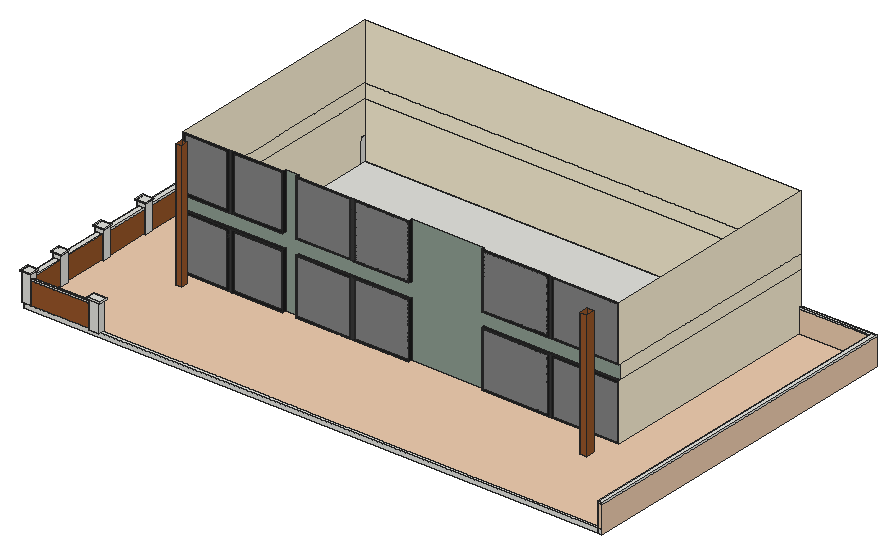
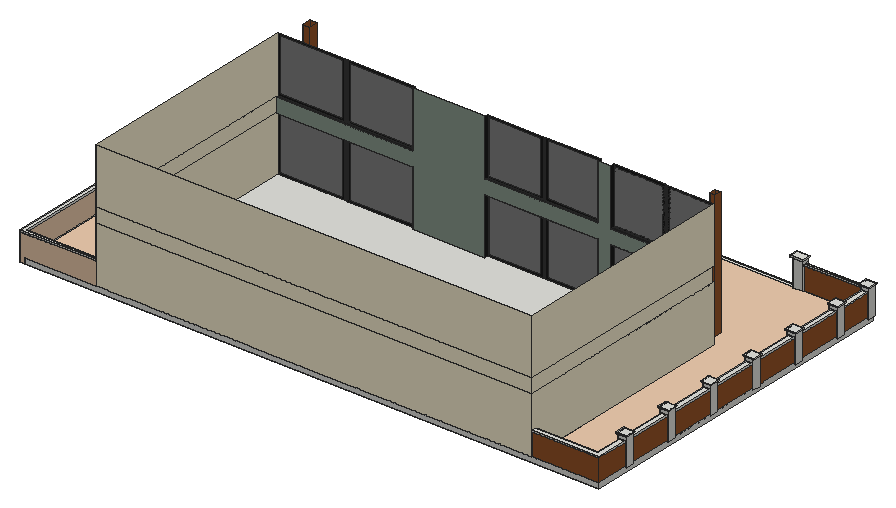
# SketchUp Ruby script. Lengths in inches.
U = 1.inch
M = Sketchup.active_model
def pt(a) = Geom::Point3d.new(a.map { |v| v * U })
def face(e, loops, mat)
  f = e.add_face(loops[0].map { |a| pt(a) })
  loops[1..].each { |l| e.add_face(l.map { |a| pt(a) }).erase! }
  f.material = f.back_material = mat if mat
  f
end
# faces: each face lists its corners as indices into pts; further lists are holes
def faces(e, pts, list, mat = nil) = list.each { |f| face(e, (f[0].is_a?(Array) ? f : [f]).map { |l| l.map { |i| pts[i] } }, mat) }
# xy, xz, yz: faces in a plane at the given z, y or x. An outline is a flat list of corners, or four numbers for a rectangle; further outlines are holes
def ring(l) = l.size == 4 ? [[l[0], l[1]], [l[2], l[1]], [l[2], l[3]], [l[0], l[3]]] : l.each_slice(2).to_a
def flat(e, list, mat, &to3) = list.each { |f| face(e, (f[0].is_a?(Array) ? f : [f]).map { |l| ring(l).map { |u, v| to3.(u, v) } }, mat) }
def xy(e, z, list, mat = nil) = flat(e, list, mat) { |x, y| [x, y, z] }
def xz(e, y, list, mat = nil) = flat(e, list, mat) { |x, z| [x, y, z] }
def yz(e, x, list, mat = nil) = flat(e, list, mat) { |y, z| [x, y, z] }
def lines(e, pts, list) = list.each { |a, b| e.add_line(pt(pts[a]), pt(pts[b])) }
# prism: a flat outline (further loops are holes) pulled along v
def prism(e, loops, v, mat = nil)
  f = face(e, loops, mat); d = Geom::Vector3d.new(v.map { |x| x * U })
  f.pushpull(f.normal.samedirection?(d) ? d.length : -d.length)
end
def box(e, o, s, mat = nil) = prism(e, [[o, [o[0] + s[0], o[1], o[2]], [o[0] + s[0], o[1] + s[1], o[2]], [o[0], o[1] + s[1], o[2]]]], [0, 0, s[2]], mat)
def at(x, y, z, deg = 0) = Geom::Transformation.translation(pt([x, y, z])) * Geom::Transformation.rotation(ORIGIN, Z_AXIS, deg.degrees)
def axes(o, x, y, z) = Geom::Transformation.new([*x, 0, *y, 0, *z, 0, *pt(o).to_a, 1])
def part(name) = M.definitions.add(name)
# library, detail: a bought-in or finely detailed component or shape, given as its bounding box
def library(name, o, s) = part(name).tap { |d| box(d.entities, o, s) }
def detail(e, o, s) = box(e.add_group.entities, o, s)
def put(e, d, t, mat = nil) = e.add_instance(d, t).tap { |i| i.material = mat if mat }
def group(e, t, mat = nil) = e.add_group.tap { |g| g.transformation = t; g.material = mat if mat }.entities
root = M.entities
M.materials.add("Generic\#5").color = [249, 239, 211]
M.materials.add("Generic\#6").color = [237, 204, 174]
M.materials.add("[Color M07]").color = [58, 58, 58]
M.materials.add("[Color M08]").color = [30, 30, 30]
M.materials.add("[Mirror 01]").color = [132, 132, 132]
M.materials.add("[Translucent Glass Corrugated]1").color = [141, 158, 145]
M.materials.add("[Wood Cherry Original]").color = [150, 85, 41]
M.materials.add("[Wood Cherry Original]1").color = [152, 86, 42]
xy(root,-14.3125,[[7.6875,8.875,1724.5,1033.625],[1724.5,8.875,1738.3125,1033.625]])
xy(root,0,[[207.01,4.0625,236.49,8.875],[3.125,8.875,7.6875,30],[7.6875,8.875,28.4375,30],[28.4375,8.875,207.01,16.875],[207.01,8.875,236.49,21.6875],
  [236.49,8.875,1724.5,16.875],[7.6875,30,23.875,122.6875],[3.125,122.6875,7.6875,146.3125],[7.6875,122.6875,28.4375,146.3125],[7.6875,146.3125,23.875,280.75],
  [1471.55,257.9375,1493.05,285.22],[3.125,280.75,7.6875,304.375],[7.6875,280.75,28.4375,304.375],[233.49,296.48,249.12,318.23],[7.6875,304.375,23.875,438.8125],
  [209.5,351.125,509.5,351.125,509.5,360,548.8125,360,548.8125,351.125,886.67,351.125,886.67,360,1103.86,360,1103.86,351.125,1513,351.125,1513,1033.625,209.5,1033.625],[3.125,438.8125,7.6875,462.4375],[7.6875,438.8125,28.4375,462.4375],[7.6875,462.4375,23.875,596.875],[3.125,596.875,7.6875,620.5],
  [7.6875,596.875,28.4375,620.5],[7.6875,620.5,23.875,754.9375],[3.125,754.9375,7.6875,778.5625],[7.6875,754.9375,28.4375,778.5625],[7.6875,778.5625,23.875,913],
  [3.125,913,7.6875,936.625],[7.6875,913,28.4375,936.625],[7.6875,936.625,23.875,1033.625],[23.875,1018.4375,209.5,1033.625]])
xy(root,0,[[[28.4375,16.875,207.01,16.875,207.01,21.6875,236.49,21.6875,236.49,16.875,1724.5,16.875,1724.5,1025.25,1513,1025.25,1513,351.125,1103.86,351.125,1103.86,360,886.67,360,886.67,351.125,548.8125,351.125,548.8125,360,509.5,360,509.5,351.125,209.5,351.125,209.5,1018.4375,23.875,1018.4375,23.875,936.625,28.4375,936.625,28.4375,913,23.875,913,23.875,778.5625,28.4375,778.5625,28.4375,754.9375,23.875,754.9375,23.875,620.5,28.4375,620.5,28.4375,596.875,23.875,596.875,23.875,462.4375,28.4375,462.4375,28.4375,438.8125,23.875,438.8125,23.875,304.375,28.4375,304.375,28.4375,280.75,23.875,280.75,23.875,146.3125,28.4375,146.3125,28.4375,122.6875,23.875,122.6875,23.875,30,28.4375,30],[1471.55,257.9375,1493.05,285.22],[233.49,296.48,249.12,318.23]],[1513,1025.25,1724.5,1033.625]],"Generic\#6")
xy(root,66.8125,[[28.4375,8.875,207.01,16.875],[1724.5,8.875,1724.5,1025.25,1513,1025.25,1513,1033.625,1738.3125,1033.625,1738.3125,8.875],[7.6875,30,23.875,122.6875],[7.6875,146.3125,23.875,280.75],[7.6875,304.375,23.875,438.8125],
  [7.6875,462.4375,23.875,596.875],[7.6875,620.5,23.875,754.9375],[7.6875,778.5625,23.875,913],[7.6875,936.625,23.875,1033.625],[23.875,1018.4375,209.5,1033.625]])
xy(root,71.3125,[[28.4375,8.875,207.01,16.875],[1724.5,8.875,1738.3125,8.875,1738.3125,1033.625,1513,1033.625,1513,1025.25,1724.5,1025.25],[7.6875,30,23.875,122.6875],[7.6875,146.3125,23.875,280.75],[7.6875,304.375,23.875,438.8125],
  [7.6875,462.4375,23.875,596.875],[7.6875,620.5,23.875,754.9375],[7.6875,778.5625,23.875,913],[7.6875,936.625,23.875,936.625,23.875,1018.4375,209.5,1018.4375,209.5,1033.625,7.6875,1033.625]])
xy(root,83.0625,[[202.95,0,241.43,4.0625],[202.95,4.0625,207.01,25.75],[207.01,4.0625,236.49,21.6875],[236.49,4.0625,241.43,21.6875],[207.01,21.6875,241.43,25.75]])
xy(root,85,[[0,5.75,3.125,33.125],[3.125,5.75,31.5625,8.875],[3.125,8.875,28.4375,30],[28.4375,8.875,31.5625,30],[3.125,30,31.5625,33.125],
  [0,119.5625,31.5625,122.6875],[0,122.6875,3.125,149.4375],[3.125,122.6875,28.4375,146.3125],[28.4375,122.6875,31.5625,149.4375],[3.125,146.3125,28.4375,149.4375],
  [0,277.625,3.125,307.5],[3.125,277.625,31.5625,280.75],[3.125,280.75,28.4375,304.375],[28.4375,280.75,31.5625,304.375],[3.125,304.375,31.5625,307.5],
  [0,435.6875,28.4375,438.8125],[28.4375,435.6875,31.5625,465.5625],[0,438.8125,3.125,465.5625],[3.125,438.8125,28.4375,462.4375],[3.125,462.4375,28.4375,465.5625],
  [0,593.75,28.4375,596.875],[28.4375,593.75,31.5625,623.625],[0,596.875,3.125,623.625],[3.125,596.875,28.4375,620.5],[3.125,620.5,28.4375,623.625],
  [0,751.8125,28.4375,754.9375],[28.4375,751.8125,31.5625,781.6875],[0,754.9375,3.125,781.6875],[3.125,754.9375,28.4375,778.5625],[3.125,778.5625,28.4375,781.6875],
  [0,909.875,28.4375,913],[28.4375,909.875,31.5625,939.75],[0,913,3.125,939.75],[3.125,913,28.4375,936.625],[3.125,936.625,28.4375,939.75]])
xy(root,87.1875,[[202.95,0,241.43,25.75],[0,5.75,31.5625,33.125],[0,119.5625,31.5625,149.4375],[0,277.625,31.5625,307.5],[0,435.6875,31.5625,465.5625],
  [0,593.75,31.5625,623.625],[0,751.8125,31.5625,781.6875],[0,909.875,31.5625,939.75]])
xy(root,168,[[209.5,351.125,347.5,360],[347.5,351.125,357.5,360],[357.5,351.125,509.5,360],[548.8125,351.125,712.74,360],[712.74,351.125,722.74,360],
  [722.74,351.125,886.67,360],[1103.86,351.125,1303.43,360],[1303.43,351.125,1313.43,360],[1313.43,351.125,1513,360]],"[Color M08]")
xy(root,210.75,[[209.5,351.125,347.5,360],[347.5,351.125,357.5,360],[357.5,351.125,509.5,360],[548.8125,351.125,712.74,360],[712.74,351.125,722.74,360],
  [722.74,351.125,886.67,360],[1103.86,351.125,1303.43,360],[1303.43,351.125,1313.43,360],[1313.43,351.125,1513,360]],"[Color M08]")
xz(root,0,[[202.95,83.0625,241.43,87.1875]])
xz(root,4.0625,[[207.01,0,236.49,83.0625]])
xz(root,5.75,[[0,85,31.5625,87.1875]])
xz(root,8.875,[[7.6875,-14.3125,1724.5,0],[1724.5,-14.3125,1738.3125,0],[3.125,0,28.4375,85],[28.4375,66.8125,207.01,71.3125],[1724.5,66.8125,1738.3125,71.3125]])
xz(root,8.875,[[1724.5,0,1738.3125,66.8125]],"Generic\#6")
xz(root,8.875,[[28.4375,0,207.01,66.8125]],"[Wood Cherry Original]")
xz(root,16.875,[[28.4375,66.8125,207.01,71.3125]])
xz(root,16.875,[[28.4375,0,207.01,66.8125]],"[Wood Cherry Original]")
xz(root,21.6875,[[207.01,0,236.49,83.0625]])
xz(root,25.75,[[202.95,83.0625,241.43,87.1875]])
xz(root,30,[[3.125,0,7.6875,66.8125],[7.6875,0,23.875,66.8125],[23.875,0,28.4375,66.8125],[3.125,66.8125,7.6875,71.3125],[7.6875,66.8125,23.875,71.3125],
  [23.875,66.8125,28.4375,71.3125],[3.125,71.3125,28.4375,85]])
xz(root,33.125,[[0,85,31.5625,87.1875]])
xz(root,119.5625,[[0,85,31.5625,87.1875]])
xz(root,122.6875,[[3.125,0,7.6875,0,7.6875,71.3125,23.875,71.3125,23.875,0,28.4375,0,28.4375,85,3.125,85],[7.6875,0,23.875,66.8125],[7.6875,66.8125,23.875,71.3125]])
xz(root,146.3125,[[3.125,0,7.6875,66.8125],[7.6875,0,23.875,66.8125],[23.875,0,28.4375,66.8125],[3.125,66.8125,7.6875,71.3125],[7.6875,66.8125,23.875,71.3125],
  [23.875,66.8125,28.4375,71.3125],[3.125,71.3125,28.4375,85]])
xz(root,149.4375,[[0,85,31.5625,87.1875]])
xz(root,257.9375,[[1471.55,0,1493.05,378.75]],"[Wood Cherry Original]")
xz(root,277.625,[[0,85,31.5625,87.1875]])
xz(root,280.75,[[3.125,0,7.6875,0,7.6875,71.3125,23.875,71.3125,23.875,0,28.4375,0,28.4375,85,3.125,85],[7.6875,0,23.875,66.8125],[7.6875,66.8125,23.875,71.3125]])
xz(root,285.22,[[1471.55,0,1493.05,378.75]],"[Wood Cherry Original]")
xz(root,296.48,[[233.49,0,249.12,378.75]],"[Wood Cherry Original]1")
xz(root,304.375,[[3.125,0,7.6875,66.8125],[7.6875,0,23.875,66.8125],[23.875,0,28.4375,66.8125],[3.125,66.8125,7.6875,71.3125],[7.6875,66.8125,23.875,71.3125],
  [23.875,66.8125,28.4375,71.3125],[3.125,71.3125,28.4375,85]])
xz(root,307.5,[[0,85,31.5625,87.1875]])
xz(root,318.23,[[233.49,0,249.12,378.75]],"[Wood Cherry Original]1")
xz(root,351.125,[[347.5,0,357.5,168],[712.74,0,722.74,168],[1303.43,0,1313.43,168],[347.5,210.75,357.5,378.75],[712.74,210.75,722.74,378.75],
  [1303.43,210.75,1313.43,378.75]],"[Color M07]")
xz(root,351.125,[[[209.5,0,347.5,168],[214.38,4.88,342.62,163.12]],[[357.5,0,509.5,168],[362.38,4.88,504.62,163.12]],[[548.8125,0,712.74,168],[553.7,4.88,707.86,163.12]],[[722.74,0,886.67,168],[727.625,4.88,881.79,163.12]],[[1103.86,0,1303.43,168],[1108.74,4.88,1298.55,163.12]],
  [[1313.43,0,1513,168],[1318.3125,4.88,1508.12,163.12]],[[209.5,210.75,347.5,378.75],[214.38,215.63,342.62,373.87]],[[357.5,210.75,509.5,378.75],[362.38,215.63,504.62,373.87]],[[548.8125,210.75,712.74,378.75],[553.7,215.63,707.86,373.87]],[[722.74,210.75,886.67,378.75],[727.625,215.63,881.79,373.87]],
  [[1103.86,210.75,1303.43,378.75],[1108.74,215.63,1298.55,373.87]],[[1313.43,210.75,1513,378.75],[1318.3125,215.63,1508.12,373.87]]],"[Color M08]")
xz(root,351.125,[[214.38,4.88,342.62,163.12],[362.38,4.88,504.62,163.12],[553.7,4.88,707.86,163.12],[727.625,4.88,881.79,163.12],[1108.74,4.88,1298.55,163.12],
  [1318.3125,4.88,1508.12,163.12],[214.38,215.63,342.62,373.87],[362.38,215.63,504.62,373.87],[553.7,215.63,707.86,373.87],[727.625,215.63,881.79,373.87],
  [1108.74,215.63,1298.55,373.87],[1318.3125,215.63,1508.12,373.87]],"[Mirror 01]")
xz(root,360,[[509.5,0,548.8125,0,548.8125,168,886.67,168,886.67,0,1103.86,0,1103.86,168,1513,168,1513,210.75,1103.86,210.75,1103.86,378.75,886.67,378.75,886.67,210.75,548.8125,210.75,548.8125,378.75,509.5,378.75,509.5,210.75,209.5,210.75,209.5,168,509.5,168]],"[Translucent Glass Corrugated]1")
xz(root,435.6875,[[0,85,31.5625,87.1875]])
xz(root,438.8125,[[3.125,0,7.6875,0,7.6875,71.3125,23.875,71.3125,23.875,0,28.4375,0,28.4375,85,3.125,85],[7.6875,0,23.875,66.8125],[7.6875,66.8125,23.875,71.3125]])
xz(root,462.4375,[[3.125,0,7.6875,66.8125],[7.6875,0,23.875,66.8125],[23.875,0,28.4375,66.8125],[3.125,66.8125,7.6875,71.3125],[7.6875,66.8125,23.875,71.3125],
  [23.875,66.8125,28.4375,71.3125],[3.125,71.3125,28.4375,85]])
xz(root,465.5625,[[0,85,31.5625,87.1875]])
xz(root,593.75,[[0,85,31.5625,87.1875]])
xz(root,596.875,[[3.125,0,7.6875,0,7.6875,71.3125,23.875,71.3125,23.875,0,28.4375,0,28.4375,85,3.125,85],[7.6875,0,23.875,66.8125],[7.6875,66.8125,23.875,71.3125]])
xz(root,620.5,[[3.125,0,7.6875,66.8125],[7.6875,0,23.875,66.8125],[23.875,0,28.4375,66.8125],[3.125,66.8125,7.6875,71.3125],[7.6875,66.8125,23.875,71.3125],
  [23.875,66.8125,28.4375,71.3125],[3.125,71.3125,28.4375,85]])
xz(root,623.625,[[0,85,31.5625,87.1875]])
xz(root,751.8125,[[0,85,31.5625,87.1875]])
xz(root,754.9375,[[3.125,0,7.6875,0,7.6875,71.3125,23.875,71.3125,23.875,0,28.4375,0,28.4375,85,3.125,85],[7.6875,0,23.875,66.8125],[7.6875,66.8125,23.875,71.3125]])
xz(root,778.5625,[[3.125,0,7.6875,66.8125],[7.6875,0,23.875,66.8125],[23.875,0,28.4375,66.8125],[3.125,66.8125,7.6875,71.3125],[7.6875,66.8125,23.875,71.3125],
  [23.875,66.8125,28.4375,71.3125],[3.125,71.3125,28.4375,85]])
xz(root,781.6875,[[0,85,31.5625,87.1875]])
xz(root,909.875,[[0,85,31.5625,87.1875]])
xz(root,913,[[3.125,0,7.6875,0,7.6875,71.3125,23.875,71.3125,23.875,0,28.4375,0,28.4375,85,3.125,85],[7.6875,0,23.875,66.8125],[7.6875,66.8125,23.875,71.3125]])
xz(root,936.625,[[3.125,0,7.6875,66.8125],[7.6875,0,23.875,66.8125],[23.875,0,28.4375,66.8125],[3.125,66.8125,7.6875,71.3125],[7.6875,66.8125,23.875,71.3125],
  [23.875,66.8125,28.4375,71.3125],[3.125,71.3125,28.4375,85]])
xz(root,939.75,[[0,85,31.5625,87.1875]])
xz(root,1018.4375,[[23.875,66.8125,209.5,71.3125]])
xz(root,1018.4375,[[23.875,0,209.5,66.8125]],"Generic\#6")
xz(root,1025.25,[[1513,66.8125,1724.5,71.3125]])
xz(root,1025.25,[[1513,0,1724.5,66.8125]],"Generic\#6")
xz(root,1033.625,[[7.6875,-14.3125,1724.5,0],[7.6875,66.8125,209.5,71.3125],[1513,66.8125,1738.3125,71.3125]])
xz(root,1033.625,[[209.5,0,1513,168],[209.5,168,1513,210.75],[209.5,210.75,1513,378.75]],"Generic\#5")
xz(root,1033.625,[[1724.5,-14.3125,1724.5,0,1513,0,1513,66.8125,1738.3125,66.8125,1738.3125,-14.3125]],"Generic\#6")
xz(root,1033.625,[[7.6875,0,209.5,66.8125]],"[Wood Cherry Original]")
yz(root,0,[[5.75,85,33.125,87.1875],[119.5625,85,149.4375,87.1875],[277.625,85,307.5,87.1875],[435.6875,85,465.5625,87.1875],[593.75,85,623.625,87.1875],
  [751.8125,85,781.6875,87.1875],[909.875,85,939.75,87.1875]])
yz(root,3.125,[[8.875,0,30,85],[122.6875,0,146.3125,85],[280.75,0,304.375,85],[438.8125,0,462.4375,85],[596.875,0,620.5,85],
  [754.9375,0,778.5625,85],[913,0,936.625,85]])
yz(root,7.6875,[[8.875,-14.3125,1033.625,0],[30,66.8125,122.6875,71.3125],[146.3125,66.8125,280.75,71.3125],[304.375,66.8125,438.8125,71.3125],[462.4375,66.8125,596.875,71.3125],
  [620.5,66.8125,754.9375,71.3125],[778.5625,66.8125,913,71.3125],[936.625,66.8125,1033.625,71.3125]])
yz(root,7.6875,[[30,0,122.6875,66.8125],[146.3125,0,280.75,66.8125],[304.375,0,438.8125,66.8125],[462.4375,0,596.875,66.8125],[620.5,0,754.9375,66.8125],
  [778.5625,0,913,66.8125],[936.625,0,1033.625,66.8125]],"[Wood Cherry Original]")
yz(root,23.875,[[30,66.8125,122.6875,71.3125],[146.3125,66.8125,280.75,71.3125],[304.375,66.8125,438.8125,71.3125],[462.4375,66.8125,596.875,71.3125],[620.5,66.8125,754.9375,71.3125],
  [778.5625,66.8125,913,71.3125],[936.625,66.8125,1018.4375,71.3125]])
yz(root,23.875,[[30,0,122.6875,66.8125],[146.3125,0,280.75,66.8125],[304.375,0,438.8125,66.8125],[462.4375,0,596.875,66.8125],[620.5,0,754.9375,66.8125],
  [778.5625,0,913,66.8125],[936.625,0,1018.4375,66.8125]],"[Wood Cherry Original]")
yz(root,28.4375,[[16.875,0,30,0,30,85,8.875,85,8.875,71.3125,16.875,71.3125],[8.875,0,16.875,66.8125],[122.6875,0,146.3125,85],[280.75,0,304.375,85],[438.8125,0,462.4375,85],
  [596.875,0,620.5,85],[754.9375,0,778.5625,85],[913,0,936.625,85],[8.875,66.8125,16.875,71.3125]])
yz(root,31.5625,[[5.75,85,33.125,87.1875],[119.5625,85,149.4375,87.1875],[277.625,85,307.5,87.1875],[435.6875,85,465.5625,87.1875],[593.75,85,623.625,87.1875],
  [751.8125,85,781.6875,87.1875],[909.875,85,939.75,87.1875]])
yz(root,202.95,[[0,83.0625,25.75,87.1875]])
yz(root,207.01,[[4.0625,0,8.875,66.8125],[8.875,0,16.875,66.8125],[16.875,0,21.6875,66.8125],[4.0625,66.8125,8.875,71.3125],[8.875,66.8125,16.875,71.3125],
  [16.875,66.8125,21.6875,71.3125],[4.0625,71.3125,21.6875,83.0625]])
yz(root,209.5,[[1018.4375,0,1033.625,66.8125]])
yz(root,209.5,[[351.125,0,351.125,168,1033.625,168,1033.625,71.3125,1018.4375,71.3125,1018.4375,0],[360,168,1033.625,210.75],[351.125,210.75,1033.625,378.75]],"Generic\#5")
yz(root,233.49,[[296.48,0,318.23,378.75]],"[Wood Cherry Original]1")
yz(root,236.49,[[4.0625,0,21.6875,83.0625]])
yz(root,241.43,[[0,83.0625,25.75,87.1875]])
yz(root,249.12,[[296.48,0,318.23,378.75]],"[Wood Cherry Original]1")
yz(root,509.5,[[351.125,0,360,168],[351.125,210.75,360,378.75]],"[Color M08]")
yz(root,548.8125,[[351.125,0,360,168],[351.125,210.75,360,378.75]],"[Color M08]")
yz(root,886.67,[[351.125,0,360,168],[351.125,210.75,360,378.75]],"[Color M08]")
yz(root,1103.86,[[351.125,0,360,168],[351.125,210.75,360,378.75]],"[Color M08]")
yz(root,1471.55,[[257.9375,0,285.22,378.75]],"[Wood Cherry Original]")
yz(root,1493.05,[[257.9375,0,285.22,378.75]],"[Wood Cherry Original]")
yz(root,1513,[[351.125,0,1025.25,0,1025.25,71.3125,1033.625,71.3125,1033.625,168,351.125,168],[360,168,1033.625,210.75],[351.125,210.75,1033.625,378.75]],"Generic\#5")
yz(root,1724.5,[[8.875,-14.3125,1033.625,0],[8.875,66.8125,1025.25,71.3125]])
yz(root,1724.5,[[8.875,0,1025.25,66.8125]],"Generic\#6")
yz(root,1738.3125,[[8.875,66.8125,1033.625,71.3125]])
yz(root,1738.3125,[[8.875,-14.3125,1033.625,66.8125]],"Generic\#6")
